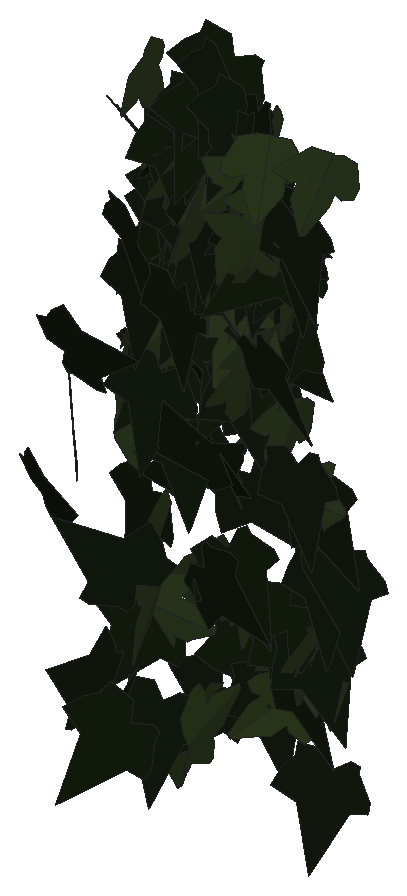
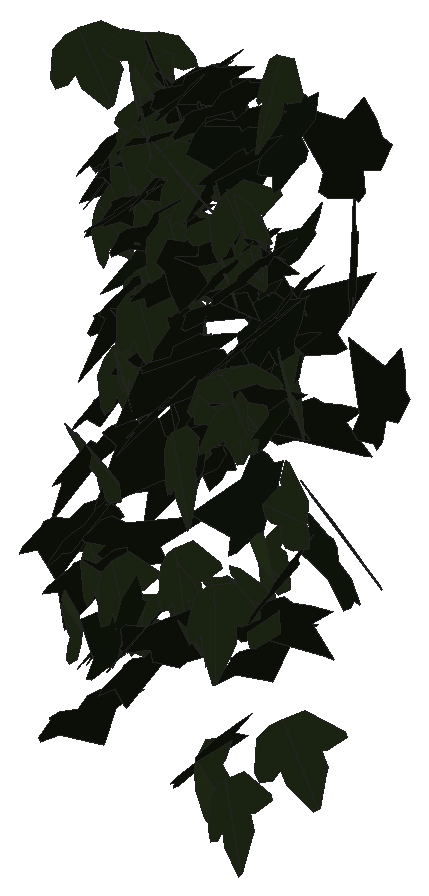
# SketchUp Ruby script. Lengths in inches.
U = 1.inch
M = Sketchup.active_model
def pt(a) = Geom::Point3d.new(a.map { |v| v * U })
def face(e, loops, mat)
  f = e.add_face(loops[0].map { |a| pt(a) })
  loops[1..].each { |l| e.add_face(l.map { |a| pt(a) }).erase! }
  f.material = f.back_material = mat if mat
  f
end
# faces: each face lists its corners as indices into pts; further lists are holes
def faces(e, pts, list, mat = nil) = list.each { |f| face(e, (f[0].is_a?(Array) ? f : [f]).map { |l| l.map { |i| pts[i] } }, mat) }
# xy, xz, yz: faces in a plane at the given z, y or x. An outline is a flat list of corners, or four numbers for a rectangle; further outlines are holes
def ring(l) = l.size == 4 ? [[l[0], l[1]], [l[2], l[1]], [l[2], l[3]], [l[0], l[3]]] : l.each_slice(2).to_a
def flat(e, list, mat, &to3) = list.each { |f| face(e, (f[0].is_a?(Array) ? f : [f]).map { |l| ring(l).map { |u, v| to3.(u, v) } }, mat) }
def xy(e, z, list, mat = nil) = flat(e, list, mat) { |x, y| [x, y, z] }
def xz(e, y, list, mat = nil) = flat(e, list, mat) { |x, z| [x, y, z] }
def yz(e, x, list, mat = nil) = flat(e, list, mat) { |y, z| [x, y, z] }
def lines(e, pts, list) = list.each { |a, b| e.add_line(pt(pts[a]), pt(pts[b])) }
# prism: a flat outline (further loops are holes) pulled along v
def prism(e, loops, v, mat = nil)
  f = face(e, loops, mat); d = Geom::Vector3d.new(v.map { |x| x * U })
  f.pushpull(f.normal.samedirection?(d) ? d.length : -d.length)
end
def box(e, o, s, mat = nil) = prism(e, [[o, [o[0] + s[0], o[1], o[2]], [o[0] + s[0], o[1] + s[1], o[2]], [o[0], o[1] + s[1], o[2]]]], [0, 0, s[2]], mat)
def at(x, y, z, deg = 0) = Geom::Transformation.translation(pt([x, y, z])) * Geom::Transformation.rotation(ORIGIN, Z_AXIS, deg.degrees)
def axes(o, x, y, z) = Geom::Transformation.new([*x, 0, *y, 0, *z, 0, *pt(o).to_a, 1])
def part(name) = M.definitions.add(name)
# library, detail: a bought-in or finely detailed component or shape, given as its bounding box
def library(name, o, s) = part(name).tap { |d| box(d.entities, o, s) }
def detail(e, o, s) = box(e.add_group.entities, o, s)
def put(e, d, t, mat = nil) = e.add_instance(d, t).tap { |i| i.material = mat if mat }
def group(e, t, mat = nil) = e.add_group.tap { |g| g.transformation = t; g.material = mat if mat }.entities
root = M.entities
M.materials.add("efeu1").color = [18, 25, 13]
M.materials.add("efeu2").color = [43, 57, 29]
c1 = part("ivyleaf_9")
p = [[1.54,2.16,1.25],[1.36,2.04,1.19],[-0.21,0.99,0.68],[-0.71,1.11,0.82],[-0.85,0.86,0.67],[-0.8,0.17,0.21],
  [-0.9,-0.01,0.1],[-0.67,-0.16,-0.02],[-0.08,-0.08,-0.05],[-0.03,-0.6,-0.4],[0.65,-0.88,-0.66],[0.83,-0.6,-0.49],
  [1.29,-0.42,-0.43],[1.8125,-0.07,-0.26],[1.21,0.44,0.15]]
faces(c1.entities,p,[[0,1,2,3,4,5,6,7,8,9,10,11,12,13,14]],"efeu1")
c2 = part("ivyleaf_10")
p = [[0,0.5,-0.03],[-0.0625,2.02,-0.43],[-0.19,2.01,-0.46],[-0.54,1.05,-0.29],[-0.52,0.625,-0.18],[-0.83,0.76,-0.28],
  [-1.16,0.64,-0.33],[-1.15,0.33,-0.24],[-0.77,-0.39,0.02],[-0.3,-0.51,0.16],[0.04,-0.48,0.23],[-0.02,2.01,-0.4375],
  [-0.06,2.01,-0.43],[0.04,-0.49,0.23],[0.67,-0.49,0.14],[1.38,0.36,-0.2],[1.375,0.51,-0.24],[0.81,0.65,-0.19],
  [0.62,0.59,-0.15],[0.6,1.09,-0.28],[0.5,1.23,-0.31]]
faces(c2.entities,p,[[0,1,2,3,4,5,6,7,8,9,10],[11,12,0,13,14,15,16,17,18,19,20]],"efeu2")
put(root,c1,axes([18.01,218.8,225.95],[-0.38782,-0.29995,0.09811],[-0.07899,-0.05823,-0.49028],[0.30555,-0.39577,-0.00222]))
put(root,c1,axes([17.53,219.53,227.71],[0.05829,0.0485,0.49422],[-0.49545,-0.02797,0.06118],[0.03358,-0.49686,0.0448]))
put(root,c1,axes([16.17,219.79,230.74],[0.12952,-0.09271,0.47395],[0.39651,-0.25971,-0.15916],[0.27569,0.41708,0.00625]))
put(root,c1,axes([16.76,219.55,224.6],[-0.29601,0.38911,-0.10473],[-0.06689,0.08069,0.48889],[0.39737,0.30344,0.00428]))
put(root,c1,axes([15.99,220.16,229.1875],[-0.00696,0.02911,0.4991],[0.05776,-0.49576,0.02972],[0.4966,0.05807,0.00354]))
put(root,c1,axes([16.57,219.95,225.52],[-0.2611,0.31013,0.29265],[-0.20532,0.20931,-0.40501],[-0.37372,-0.33167,0.01805]))
put(root,c1,axes([15.13,220.58,227.78],[0.06236,-0.15882,0.46999],[0.26382,-0.39054,-0.16697],[0.42013,0.26881,0.03509]))
put(root,c1,axes([17.4375,221.27,227.08],[0.05167,-0.05614,-0.49414],[0.46264,0.18771,0.02705],[0.18248,-0.46001,0.07134]))
put(root,c1,axes([16.32,221.67,224.41],[-0.0803,-0.4933,0.01428],[-0.00209,-0.01413,-0.4998],[0.49351,-0.08033,0.00021]))
put(root,c2,axes([15.9375,221.95,225.88],[0.1331,-0.29106,0.38414],[0.21732,-0.31947,-0.31735],[0.43018,0.25144,0.04146]))
put(root,c2,axes([17.22,221.29,224.46],[0.01795,0.11002,-0.48741],[0.09091,0.47887,0.11144],[0.49134,-0.09262,-0.00281]))
put(root,c2,axes([16.72,221.59,231.78],[0.18428,-0.43036,0.1756],[-0.07054,0.16081,0.46815],[-0.45942,-0.19732,-0.00145]))
put(root,c1,axes([16.24,222.08,230.64],[0.11739,-0.46891,0.12782],[0.01286,-0.12846,-0.48305],[0.48585,0.1167,-0.0181]))
put(root,c1,axes([15.8,222.28,229.1],[-0.09952,-0.48586,0.06354],[-0.00074,-0.06468,-0.4958],[0.48999,-0.09878,0.01216]))
put(root,c1,axes([17.24,222.02,226.98],[0.08836,-0.42972,-0.23986],[-0.00607,0.24272,-0.43709],[0.49209,0.08015,0.03768]))
put(root,c1,axes([15.74,222.31,225.36],[-0.39193,-0.3037,0.0645],[-0.05184,-0.03841,-0.49582],[0.30611,-0.39534,-0.00138]))
put(root,c1,axes([16.52,222.15,227.84],[0.33226,0.09963,0.3601],[-0.36381,-0.02348,0.34218],[0.0851,-0.48941,0.05689]))
put(root,c2,axes([17.51,222.1,231.9375],[-0.40781,-0.11361,0.26606],[-0.24135,-0.11993,-0.42115],[0.15951,-0.47192,0.04298]))
put(root,c1,axes([16.24,222.33,228.46],[-0.05356,-0.49108,-0.07725],[0.00516,0.07715,-0.49399],[0.4971,-0.05372,-0.0032]))
put(root,c1,axes([17.61,222.18,230.16],[0.33901,-0.36575,-0.03609],[-0.00895,0.04086,-0.49825],[0.36741,0.33847,0.02116]))
put(root,c1,axes([16.38,222.53,231.72],[0.05817,-0.45148,0.20683],[0.04675,-0.20234,-0.45483],[0.4944,0.07225,0.01868]))
put(root,c2,axes([17.04,222.53,232.47],[-0.10013,-0.2308,0.4321],[-0.1677,-0.39823,-0.25157],[0.46027,-0.1953,0.00234]))
put(root,c2,axes([15.29,222.34,223.72],[-0.29544,-0.36154,0.1789],[-0.11798,-0.13461,-0.46686],[0.38574,-0.31807,-0.00577]))
put(root,c2,axes([15.78,222.31,225.49],[-0.03205,-0.07763,-0.4929],[0.47599,-0.15292,-0.00687],[-0.14969,-0.46967,0.0837]))
put(root,c2,axes([17.57,222.37,233.18],[0.46165,0.19138,-0.01588],[-0.01617,-0.00246,-0.49973],[-0.19136,0.46192,0.00392]))
put(root,c1,axes([15.03,222.67,230.98],[0.09686,-0.3894,0.29831],[0.11466,-0.27767,-0.39969],[0.47694,0.14584,0.03551]))
put(root,c1,axes([17.7,222.68,231.52],[-0.41309,-0.22779,0.16573],[-0.12389,-0.11728,-0.47],[0.25299,-0.42937,0.04045]))
put(root,c2,axes([17.81,222.64,224.67],[0.22486,0.17823,-0.40948],[-0.31702,-0.2592,-0.28691],[-0.31454,0.38865,-0.00356]))
put(root,c2,axes([17.42,222.6875,232.25],[-0.12907,-0.38796,0.28781],[0.01559,-0.30109,-0.39887],[0.4828,-0.09399,0.08982]))
put(root,c1,axes([15.16,222.75,230.27],[0.02325,-0.47249,0.16191],[0.00094,-0.16204,-0.47301],[0.49946,0.0223,-0.00664]))
put(root,c1,axes([16.42,222.6875,227.83],[0.12774,-0.1961,0.44184],[0.24422,-0.36822,-0.23403],[0.41718,0.2756,0.00172]))
put(root,c1,axes([17.98,222.67,225.79],[-0.277,-0.35102,-0.22373],[-0.13625,-0.17747,0.44715],[-0.39332,0.30869,0.00267]))
put(root,c1,axes([14.99,222.53,232.78],[0.40829,-0.26345,0.11788],[0.10096,-0.06094,-0.48589],[0.27038,0.42057,0.00344]))
put(root,c2,axes([17.44,222.59,231.5],[0.05599,-0.49463,0.04697],[0.00724,-0.04645,-0.49779],[0.4968,0.05642,0.00196]))
put(root,c2,axes([15.36,222.75,226.52],[0.09899,-0.29876,-0.38851],[0.22412,-0.32489,0.30695],[-0.43586,-0.23491,0.06959]))
put(root,c2,axes([17.09,222.55,229.49],[-0.05356,-0.49553,-0.03982],[0.00597,0.03941,-0.49841],[0.49709,-0.05386,0.00169]))
put(root,c1,axes([17.85,222.74,228.18],[0.08136,-0.49321,-0.01129],[-0.0013,0.01123,-0.49987],[0.49333,0.08137,0.00054]))
put(root,c1,axes([15.875,222.72,232.79],[-0.13474,-0.46499,-0.125],[0.05391,0.11442,-0.48374],[0.47848,-0.14383,0.0193]))
put(root,c2,axes([18.35,222.73,233.05],[-0.30476,-0.3439,0.19711],[-0.02088,-0.23436,-0.44118],[0.39583,-0.27714,0.12849]))
put(root,c1,axes([15.22,222.85,229.77],[-0.17489,-0.10888,0.45559],[0.22613,-0.44551,-0.01967],[0.41022,0.19917,0.20507]))
put(root,c1,axes([17.78,222.76,231.99],[0.12763,-0.48306,-0.01895],[-0.00474,0.01835,-0.49964],[0.48341,0.12772,0.00011]))
put(root,c2,axes([18.14,222.74,225.5625],[0.07794,-0.48794,0.07641],[0.02386,-0.07355,-0.49399],[0.49331,0.08065,0.01181]))
put(root,c1,axes([16.98,222.67,232.8125],[-0.45649,0.14375,0.14476],[-0.13658,0.0482,-0.47856],[-0.15154,-0.47646,-0.00474]))
put(root,c2,axes([15.9,222.69,232.25],[-0.00862,-0.49985,-0.00884],[0.00022,0.00884,-0.49992],[0.49993,-0.00863,0.00007]))
put(root,c2,axes([16.14,222.9,230.66],[-0.15523,0.21569,-0.42353],[0.17037,-0.39069,-0.26141],[-0.44371,-0.22548,0.0478]))
put(root,c1,axes([17.65,222.91,231.62],[0.11702,-0.47166,0.11765],[0.0131,-0.11791,-0.48572],[0.48594,0.11676,-0.01523]))
put(root,c1,axes([16.21,222.97,233.17],[-0.25228,-0.43025,0.03524],[-0.01004,-0.03496,-0.49868],[0.43157,-0.25232,0.009]))
put(root,c2,axes([16.9,222.76,230.09],[0.46455,0.11668,-0.14346],[-0.13836,-0.03802,-0.47897],[-0.12268,0.48471,-0.00304]))
put(root,c1,axes([17.22,222.41,232.04],[0.01041,-0.03802,-0.49844],[0.01095,0.49845,-0.03779],[0.49977,-0.01013,0.01121]))
put(root,c2,axes([17.34,222.55,232.625],[-0.10122,0.0981,-0.47972],[-0.40244,0.26237,0.13857],[0.27892,0.41417,0.02584]))
put(root,c1,axes([18.21,222.99,223.42],[-0.14368,-0.47875,0.01229],[-0.0031,-0.0119,-0.49985],[0.4789,-0.14372,0.00045]))
put(root,c2,axes([17.73,222.8125,225.4],[0.00436,-0.49785,0.04611],[0.00069,-0.0461,-0.49787],[0.49998,0.0044,0.00028]))
put(root,c1,axes([18.11,222.79,225.49],[0.00887,-0.44732,-0.22323],[0.02418,0.22338,-0.44667],[0.49934,-0.00287,0.02559]))
put(root,c1,axes([17.67,222.81,224.9],[0.27095,-0.41589,-0.06021],[-0.02747,0.05396,-0.49632],[0.41932,0.27226,0.00639]))
put(root,c1,axes([16.79,222.94,231.89],[0.10522,-0.48812,0.02577],[0.00444,-0.0254,-0.49933],[0.48878,0.10531,-0.00101]))
put(root,c2,axes([15.27,222.59,233.63],[0.04909,-0.43177,-0.24732],[0.07013,0.25204,-0.4261],[0.49262,0.00715,0.0853]))
put(root,c1,axes([16.98,222.92,233.28],[-0.32038,0.0155,-0.38356],[0.38034,-0.05484,-0.3199],[-0.05199,-0.49674,0.02335]))
put(root,c1,axes([16.15,223.14,230.86],[-0.245,-0.38858,0.19744],[-0.01306,-0.21985,-0.44888],[0.43566,-0.22511,0.09758]))
put(root,c1,axes([15.97,223.04,233.13],[-0.11169,-0.48693,0.02069],[-0.00528,-0.02001,-0.49957],[0.48734,-0.11182,-0.00067]))
put(root,c2,axes([17.22,222.81,229.93],[-0.12553,-0.48398,-0.00192],[0.00065,0.00182,-0.5],[0.48398,-0.12553,0.00017]))
put(root,c1,axes([16.61,223.13,233.15],[-0.16167,-0.45256,0.13803],[-0.02779,-0.13653,-0.48019],[0.47233,-0.16294,0.01899]))
put(root,c1,axes([15.86,223.14,230.31],[-0.21221,-0.43504,0.12532],[-0.013,-0.13249,-0.48195],[0.45255,-0.20781,0.04492]))
put(root,c1,axes([17.17,222.95,224.52],[0.05004,-0.4882,-0.09568],[0.00177,0.09634,-0.49063],[0.49749,0.04876,0.01137]))
put(root,c1,axes([15,222.83,229.07],[0.39645,-0.3044,0.01301],[0.01409,-0.00301,-0.49979],[0.30435,0.39665,0.00619]))
put(root,c2,axes([14.89,222.89,229.59],[0.25969,-0.42722,0.00646],[0.00337,-0.00551,-0.49996],[0.42726,0.25971,0.00002]))
put(root,c2,axes([17.52,223.03,228.78],[-0.05082,-0.44937,0.21326],[0.07131,-0.21874,-0.44392],[0.49227,-0.01471,0.08633]))
put(root,c1,axes([16.86,222.93,229.15],[-0.06324,-0.45243,-0.20325],[0.07294,0.19418,-0.45494],[0.49059,-0.08719,0.04144]))
put(root,c2,axes([17.14,222.82,231.16],[0.01443,-0.49387,-0.07672],[0.00253,0.07682,-0.49406],[0.49979,0.01387,0.00472]))
put(root,c1,axes([17.11,223.08,231.42],[-0.16895,-0.46958,-0.0308],[0.00519,0.03086,-0.49902],[0.47056,-0.16894,-0.00555]))
put(root,c2,axes([17.27,223.02,232.02],[-0.10705,-0.45916,0.16647],[-0.0192,-0.16633,-0.47113],[0.48803,-0.10726,0.01798]))
put(root,c1,axes([16.51,223.21,229.31],[-0.22854,-0.43188,0.10607],[-0.03204,-0.10295,-0.48824],[0.44356,-0.22996,0.01938]))
put(root,c1,axes([17.02,222.78,227.73],[-0.07403,-0.20008,-0.4522],[0.16413,0.42138,-0.21331],[0.46645,-0.18003,0.00329]))
put(root,c1,axes([15.45,223.2,228.99],[-0.37377,-0.31914,0.0919],[-0.06768,-0.06226,-0.49147],[0.32514,-0.37983,0.00334]))
put(root,c1,axes([14.83,223.29,226.49],[-0.01585,-0.39706,0.30347],[-0.01098,-0.30327,-0.39737],[0.49963,-0.01927,0.0009]))
put(root,c1,axes([17.22,223.28,232],[-0.2942,-0.30184,0.26896],[-0.16723,-0.21198,-0.42083],[0.36808,-0.33757,0.02377]))
put(root,c1,axes([15.82,222.67,232.58],[0.03719,0.49846,0.0123],[-0.00235,0.01251,-0.49984],[-0.49861,0.03712,0.00327]))
put(root,c1,axes([15.47,223.12,231.24],[-0.48502,-0.10659,-0.05825],[0.05817,0.00665,-0.49656],[0.10663,-0.48846,0.00595]))
put(root,c2,axes([17.6,223.2,231.03],[0.05717,-0.40266,0.29086],[0.1294,-0.2706,-0.40004],[0.47957,0.12101,0.07327]))
put(root,c2,axes([16.55,223.01,226.09],[-0.00607,-0.49996,0.00257],[-0.0004,-0.00256,-0.49999],[0.49996,-0.00607,-0.00037]))
put(root,c1,axes([17.35,223.35,231.2],[-0.19039,-0.40661,0.22005],[0.01158,-0.2421,-0.43733],[0.46219,-0.16143,0.10161]))
put(root,c2,axes([16.9,223.22,232.39],[-0.15381,-0.33581,0.33701],[-0.10671,-0.32081,-0.36837],[0.46363,-0.18524,0.02702]))
put(root,c2,axes([15.84,223.05,231.24],[0.24169,-0.43764,-0.00735],[-0.00818,0.00388,-0.49992],[0.43763,0.24177,-0.00529]))
put(root,c1,axes([16.15,223.38,233.43],[-0.10785,-0.43557,0.22057],[0.0147,-0.22868,-0.4444],[0.48801,-0.08937,0.06213]))
put(root,c2,axes([16.87,222.99,232.57],[-0.48,-0.02966,-0.13681],[0.1391,-0.04597,-0.47806],[0.01578,-0.497,0.05238]))
put(root,c1,axes([15.0625,222.96,230.24],[0.27683,-0.35365,-0.21976],[-0.00448,0.26136,-0.42623],[0.41635,0.23796,0.14153]))
put(root,c1,axes([17.17,223.34,229.88],[-0.20895,-0.45165,0.04853],[-0.00299,-0.05204,-0.49728],[0.45424,-0.2081,0.01905]))
put(root,c1,axes([17.89,223.29,226.39],[0.04908,-0.49386,0.06078],[-0.00312,-0.06138,-0.49621],[0.49758,0.04833,-0.0091]))
put(root,c1,axes([16.46,223.13,230.59],[0.05776,-0.46912,-0.16307],[0.01455,0.1657,-0.47152],[0.49644,0.04973,0.03279]))
put(root,c2,axes([16.75,222.92,225.74],[0.26553,-0.17941,-0.3838],[-0.29637,0.24501,-0.31958],[0.30275,0.39722,0.02377]))
put(root,c2,axes([18.4,222.875,224.53],[0.26994,-0.2734,0.31998],[-0.2217,0.23075,0.38419],[-0.35775,-0.34929,0.00335]))
put(root,c1,axes([15.5,222.99,232.53],[0.19494,-0.36649,-0.27871],[-0.03085,0.29159,-0.405],[0.4594,0.1751,0.09107]))
put(root,c2,axes([16.5,223.11,227.86],[0.09333,-0.48915,-0.04496],[-0.00912,0.04404,-0.49797],[0.49113,0.09377,-0.0007]))
put(root,c2,axes([14.53,223.13,227.61],[0.03153,-0.01755,0.4987],[0.49892,0.01051,-0.03118],[-0.00938,0.49958,0.01818]))
put(root,c1,axes([15.875,223.49,223.7],[-0.14208,-0.37878,0.29383],[-0.03701,-0.29688,-0.40061],[0.47796,-0.13558,0.05632]))
put(root,c1,axes([17.3,223.3125,224.95],[0.22099,-0.35748,0.27088],[0.15852,-0.22023,-0.41996],[0.41956,0.2715,0.016]))
put(root,c1,axes([16.9,223.41,225.17],[0.03503,-0.45737,0.19896],[0.03313,-0.19688,-0.45841],[0.49767,0.0453,0.01651]))
put(root,c2,axes([15.58,223.125,229.15],[-0.30697,-0.39206,0.04535],[-0.03214,-0.03243,-0.49791],[0.39337,-0.3086,-0.00529]))
put(root,c2,axes([17.2,223.23,229.27],[0.09535,-0.48693,0.06174],[0.00315,-0.06228,-0.4961],[0.49081,0.09499,-0.00881]))
put(root,c1,axes([16.87,223.15,224.86],[-0.40308,-0.29566,-0.01058],[-0.003,-0.0138,0.4998],[-0.29583,0.40298,0.00936]))
put(root,c1,axes([16.73,223.42,231.28],[-0.1736,-0.4673,0.03863],[-0.00986,-0.03755,-0.49849],[0.46879,-0.17384,0.00382]))
put(root,c2,axes([15.58,223.1875,223.1],[-0.01517,-0.49973,-0.00652],[0.00002,0.00652,-0.49996],[0.49977,-0.01516,-0.00017]))
put(root,c1,axes([15.36,223.38,231.2],[0.04687,-0.49582,0.04435],[0.00962,-0.04364,-0.498],[0.49771,0.04754,0.00545]))
put(root,c2,axes([17.08,223.2,232.96],[0.2967,-0.40022,-0.04234],[-0.01042,0.04495,-0.49787],[0.40232,0.29632,0.01833]))
put(root,c1,axes([15.83,223.45,231.13],[-0.37014,-0.32668,0.07923],[-0.06227,-0.04918,-0.49366],[0.33033,-0.37532,-0.00428]))
put(root,c1,axes([16.41,222.85,229.32],[0.36987,0.30197,0.14834],[0.10786,0.1024,-0.47737],[-0.31869,0.38513,0.01061]))
put(root,c1,axes([15.05,223.26,227.68],[0.35973,-0.28683,0.19576],[0.15812,-0.11565,-0.46002],[0.30917,0.39288,0.0075]))
put(root,c1,axes([16.0625,223.51,233.62],[-0.27056,-0.41005,0.09305],[-0.01443,-0.10153,-0.48937],[0.42023,-0.26749,0.0431]))
put(root,c2,axes([15.79,223.42,223.53],[0.15356,-0.40629,0.24768],[0.10038,-0.22674,-0.43418],[0.46513,0.18307,0.01193]))
put(root,c1,axes([16.58,223.27,232.27],[-0.46942,0.1684,-0.03591],[0.02776,-0.0289,-0.49839],[-0.16994,-0.4699,0.01778]))
put(root,c2,axes([17.19,223.36,229.03],[0.27166,-0.3893,0.15699],[0.10719,-0.11646,-0.47428],[0.40585,0.29134,0.02019]))
put(root,c2,axes([16.15,223.14,232.25],[-0.41984,-0.18697,-0.19691],[0.20056,0.03091,-0.45697],[0.18306,-0.46269,0.04904]))
put(root,c2,axes([15.82,223.18,225.87],[-0.09605,-0.48342,-0.08416],[0.01316,0.08319,-0.49286],[0.49051,-0.09689,-0.00325]))
put(root,c2,axes([17.5,223.38,227.32],[0.00788,-0.19212,-0.46155],[0.4,-0.27448,0.12108],[-0.2999,-0.37114,0.14937]))
put(root,c1,axes([17.22,223.02,229.97],[0.18206,-0.25642,-0.38872],[-0.16723,0.35353,-0.31153],[0.43461,0.24344,0.04296]))
put(root,c1,axes([15.11,223.6,231.12],[-0.1718,-0.39601,0.25232],[-0.02035,-0.26214,-0.42528],[0.46912,-0.1564,0.07396]))
put(root,c2,axes([15.49,223.3,229.29],[0.37256,0.26191,-0.20641],[-0.18209,-0.09949,-0.45491],[-0.27936,0.41413,0.02125]))
put(root,c2,axes([16.94,223.32,229.95],[-0.08217,-0.48578,0.08522],[-0.01176,-0.08444,-0.49268],[0.49306,-0.08297,0.00245]))
put(root,c1,axes([16.1,223.38,231.19],[-0.22645,0.27411,-0.35155],[0.10537,-0.35022,-0.34095],[-0.43315,-0.2285,0.10085]))
put(root,c2,axes([15.37,223.34,229],[0.09582,0.43985,-0.2176],[-0.06169,-0.20915,-0.44994],[-0.48684,0.11308,0.01418]))
put(root,c2,axes([16.36,223.375,231.24],[-0.14163,-0.45555,0.1497],[0.01387,-0.15993,-0.47353],[0.47932,-0.12998,0.05794]))
put(root,c1,axes([17.79,223.21,227.54],[0.17924,-0.40325,-0.23509],[-0.0882,0.21803,-0.44123],[0.45836,0.19964,0.00703]))
put(root,c2,axes([15.36,223.27,231.93],[0.44571,-0.21541,-0.07032],[-0.05934,0.0388,-0.49495],[0.21869,0.44955,0.00902]))
put(root,c1,axes([18.09,223.36,226.41],[-0.04031,-0.47303,-0.15691],[0.00207,0.15726,-0.47462],[0.49837,-0.03891,-0.01072]))
put(root,c2,axes([15.34,223.41,231.97],[-0.06665,-0.46575,0.16921],[0.00227,-0.17102,-0.46984],[0.49553,-0.06186,0.02491]))
put(root,c2,axes([15.49,223.2,231.37],[-0.41786,-0.09426,-0.2579],[0.26308,-0.0029,-0.42519],[0.07866,-0.49103,0.05201]))
put(root,c1,axes([16.5,223.27,228.73],[0.23008,-0.41632,-0.15408],[-0.00622,0.17051,-0.46999],[0.44387,0.21819,0.07328]))
